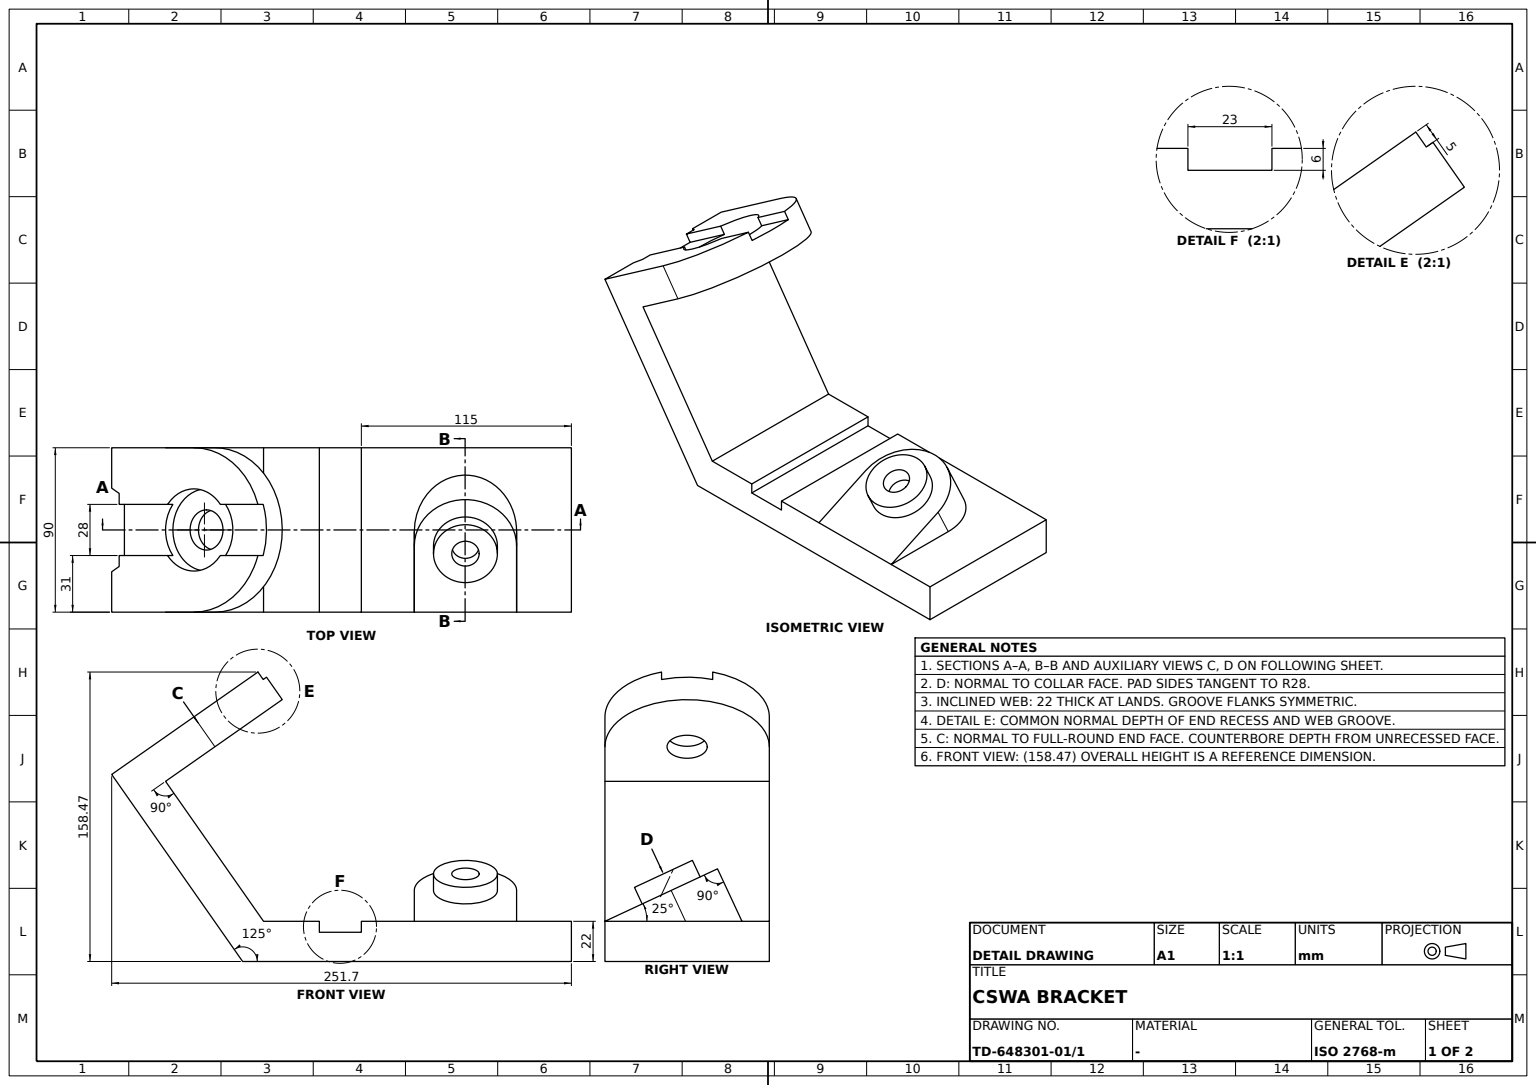
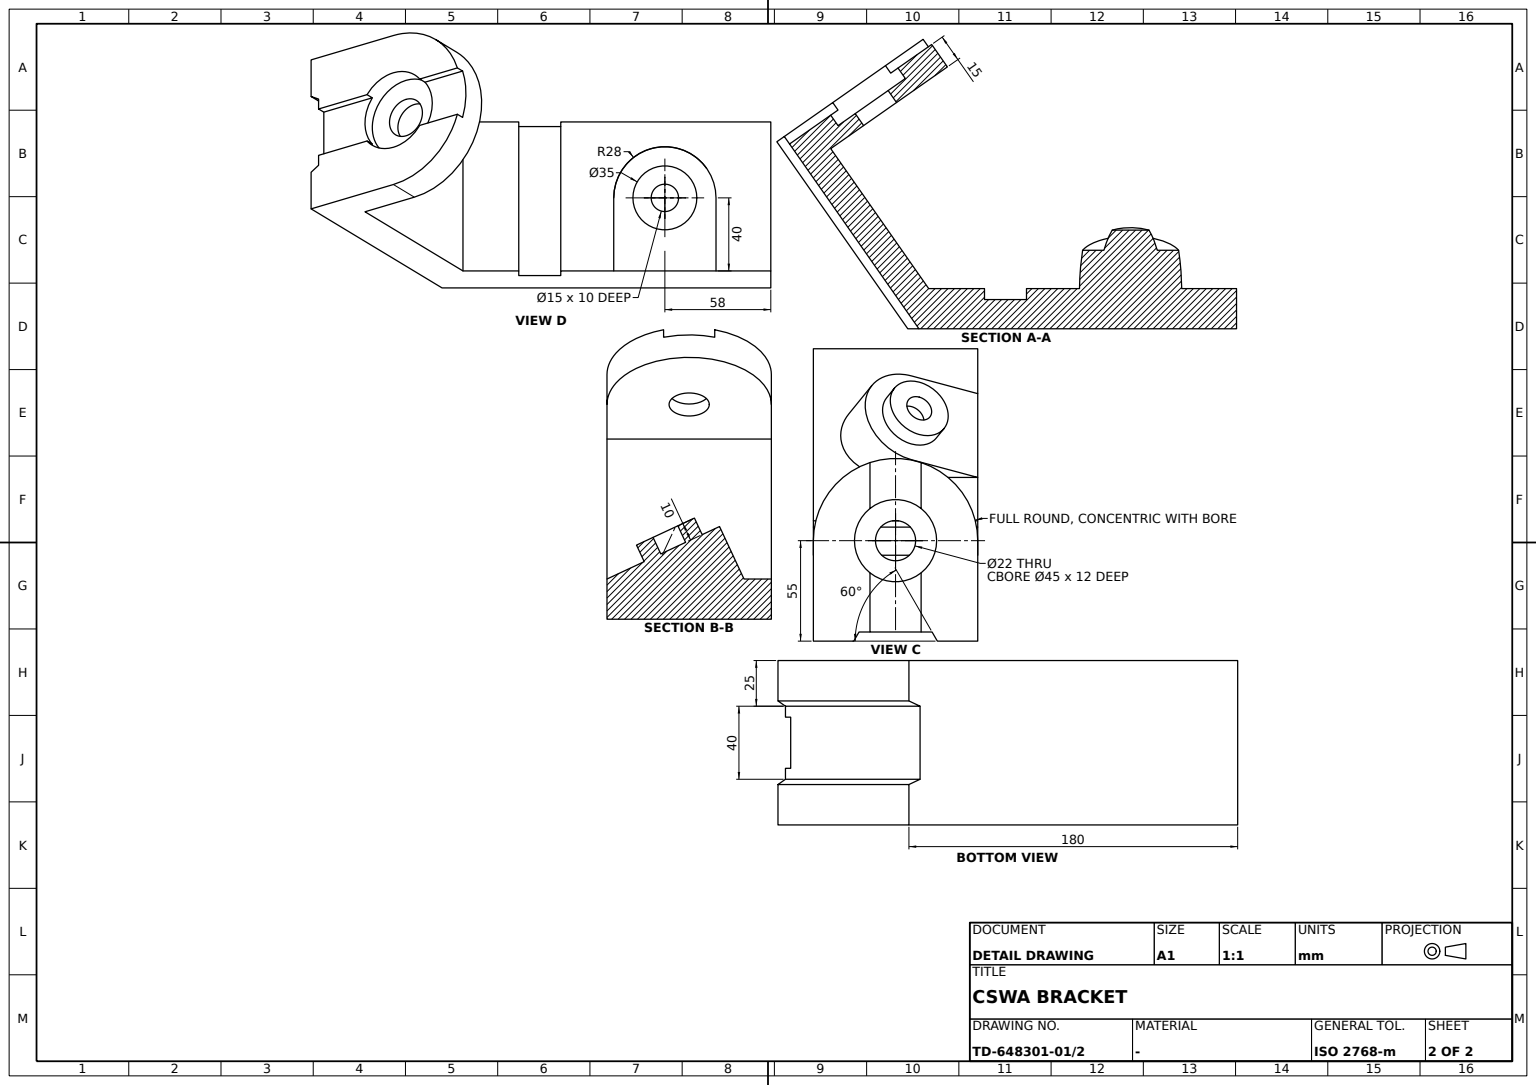
ISO-10303-21;
HEADER;
FILE_DESCRIPTION((''),'2;1');
FILE_NAME('','',(''),(''),'','','');
FILE_SCHEMA(('AUTOMOTIVE_DESIGN'));
ENDSEC;
DATA;
#1=APPLICATION_CONTEXT('');
#2=PRODUCT_CONTEXT('',#1,'mechanical');
#3=PRODUCT('','','',(#2));
#4=PRODUCT_DEFINITION_FORMATION('','',#3);
#5=PRODUCT_DEFINITION_CONTEXT('',#1,'design');
#6=PRODUCT_DEFINITION('','',#4,#5);
#7=PRODUCT_DEFINITION_SHAPE('','',#6);
#8=(LENGTH_UNIT()NAMED_UNIT(*)SI_UNIT(.MILLI.,.METRE.));
#9=(NAMED_UNIT(*)PLANE_ANGLE_UNIT()SI_UNIT($,.RADIAN.));
#10=(NAMED_UNIT(*)SI_UNIT($,.STERADIAN.)SOLID_ANGLE_UNIT());
#11=UNCERTAINTY_MEASURE_WITH_UNIT(LENGTH_MEASURE(1.E-05),#8,'distance_accuracy_value','');
#12=(GEOMETRIC_REPRESENTATION_CONTEXT(3)GLOBAL_UNCERTAINTY_ASSIGNED_CONTEXT((#11))GLOBAL_UNIT_ASSIGNED_CONTEXT((#8,#9,#10))REPRESENTATION_CONTEXT('',''));
#13=CARTESIAN_POINT('',(14.,11.25671,154.374984));
#14=VERTEX_POINT('',#13);
#15=CARTESIAN_POINT('',(-14.,11.25671,154.374984));
#16=VERTEX_POINT('',#15);
#17=CARTESIAN_POINT('',(0.,-23.77581,129.844949));
#18=DIRECTION('',(0.,-0.573576436,0.819152044));
#19=DIRECTION('',(1.,0.,0.));
#20=AXIS2_PLACEMENT_3D('',#17,#18,#19);
#21=CIRCLE('',#20,45.);
#22=EDGE_CURVE('',#14,#16,#21,.T.);
#23=ORIENTED_EDGE('',*,*,#22,.F.);
#24=CARTESIAN_POINT('',(14.,8.388827,158.470744));
#25=VERTEX_POINT('',#24);
#26=CARTESIAN_POINT('',(14.,9.822768,156.422864));
#27=DIRECTION('',(0.,0.573576436,-0.819152044));
#28=VECTOR('',#27,1000.);
#29=LINE('',#26,#28);
#30=EDGE_CURVE('',#25,#14,#29,.T.);
#31=ORIENTED_EDGE('',*,*,#30,.F.);
#32=CARTESIAN_POINT('',(45.,-26.643692,133.94071));
#33=VERTEX_POINT('',#32);
#34=CARTESIAN_POINT('',(0.,-26.643692,133.94071));
#35=AXIS2_PLACEMENT_3D('',#34,#18,#19);
#36=CIRCLE('',#35,45.);
#37=EDGE_CURVE('',#33,#25,#36,.T.);
#38=ORIENTED_EDGE('',*,*,#37,.F.);
#39=CARTESIAN_POINT('',(45.,-15.172163,117.557669));
#40=VERTEX_POINT('',#39);
#41=CARTESIAN_POINT('',(45.,-20.907928,125.749189));
#42=VECTOR('',#18,1000.);
#43=LINE('',#41,#42);
#44=EDGE_CURVE('',#40,#33,#43,.T.);
#45=ORIENTED_EDGE('',*,*,#44,.F.);
#46=CARTESIAN_POINT('',(-45.,-15.172163,117.557669));
#47=VERTEX_POINT('',#46);
#48=CARTESIAN_POINT('',(0.,-15.172163,117.557669));
#49=AXIS2_PLACEMENT_3D('',#48,#18,#19);
#50=CIRCLE('',#49,45.);
#51=EDGE_CURVE('',#40,#47,#50,.T.);
#52=ORIENTED_EDGE('',*,*,#51,.T.);
#53=CARTESIAN_POINT('',(-45.,-26.643692,133.94071));
#54=VERTEX_POINT('',#53);
#55=CARTESIAN_POINT('',(-45.,-20.907928,125.749189));
#56=LINE('',#55,#42);
#57=EDGE_CURVE('',#47,#54,#56,.T.);
#58=ORIENTED_EDGE('',*,*,#57,.T.);
#59=CARTESIAN_POINT('',(-14.,8.388827,158.470744));
#60=VERTEX_POINT('',#59);
#61=EDGE_CURVE('',#60,#54,#36,.T.);
#62=ORIENTED_EDGE('',*,*,#61,.F.);
#63=CARTESIAN_POINT('',(-14.,9.822768,156.422864));
#64=LINE('',#63,#28);
#65=EDGE_CURVE('',#60,#16,#64,.T.);
#66=ORIENTED_EDGE('',*,*,#65,.T.);
#67=EDGE_LOOP('',(#23,#31,#38,#45,#52,#58,#62,#66));
#68=FACE_OUTER_BOUND('',#67,.T.);
#69=CARTESIAN_POINT('',(0.,-20.907928,125.749189));
#70=AXIS2_PLACEMENT_3D('',#69,#27,#19);
#71=CYLINDRICAL_SURFACE('',#70,45.);
#72=ADVANCED_FACE('',(#68),#71,.T.);
#73=CARTESIAN_POINT('',(-14.,-38.204284,119.742023));
#74=VERTEX_POINT('',#73);
#75=CARTESIAN_POINT('',(14.,-38.204284,119.742023));
#76=VERTEX_POINT('',#75);
#77=CIRCLE('',#20,22.5);
#78=EDGE_CURVE('',#74,#76,#77,.T.);
#79=ORIENTED_EDGE('',*,*,#78,.F.);
#80=CARTESIAN_POINT('',(-14.,-64.733412,101.166127));
#81=VERTEX_POINT('',#80);
#82=CARTESIAN_POINT('',(-14.,-51.468848,110.454075));
#83=DIRECTION('',(0.,-0.819152044,-0.573576436));
#84=VECTOR('',#83,1000.);
#85=LINE('',#82,#84);
#86=EDGE_CURVE('',#74,#81,#85,.T.);
#87=ORIENTED_EDGE('',*,*,#86,.T.);
#88=CARTESIAN_POINT('',(14.,-64.733412,101.166127));
#89=VERTEX_POINT('',#88);
#90=CARTESIAN_POINT('',(0.,-64.733412,101.166127));
#91=VECTOR('',#19,1000.);
#92=LINE('',#90,#91);
#93=EDGE_CURVE('',#81,#89,#92,.T.);
#94=ORIENTED_EDGE('',*,*,#93,.T.);
#95=CARTESIAN_POINT('',(14.,-51.468848,110.454075));
#96=DIRECTION('',(0.,0.819152044,0.573576436));
#97=VECTOR('',#96,1000.);
#98=LINE('',#95,#97);
#99=EDGE_CURVE('',#89,#76,#98,.T.);
#100=ORIENTED_EDGE('',*,*,#99,.T.);
#101=EDGE_LOOP('',(#79,#87,#94,#100));
#102=FACE_OUTER_BOUND('',#101,.T.);
#103=CARTESIAN_POINT('',(0.,-68.829172,98.298245));
#104=AXIS2_PLACEMENT_3D('',#103,#18,#19);
#105=PLANE('',#104);
#106=ADVANCED_FACE('',(#102),#105,.T.);
#107=CARTESIAN_POINT('',(11.,-15.172163,117.557669));
#108=VERTEX_POINT('',#107);
#109=CARTESIAN_POINT('',(11.,-19.760775,124.110885));
#110=VERTEX_POINT('',#109);
#111=CARTESIAN_POINT('',(11.,-17.466469,120.834277));
#112=LINE('',#111,#42);
#113=EDGE_CURVE('',#108,#110,#112,.T.);
#114=ORIENTED_EDGE('',*,*,#113,.F.);
#115=CARTESIAN_POINT('',(-11.,-15.172163,117.557669));
#116=VERTEX_POINT('',#115);
#117=AXIS2_PLACEMENT_3D('',#48,#27,#19);
#118=CIRCLE('',#117,11.);
#119=EDGE_CURVE('',#108,#116,#118,.T.);
#120=ORIENTED_EDGE('',*,*,#119,.T.);
#121=CARTESIAN_POINT('',(-11.,-19.760775,124.110885));
#122=VERTEX_POINT('',#121);
#123=CARTESIAN_POINT('',(-11.,-17.466469,120.834277));
#124=LINE('',#123,#42);
#125=EDGE_CURVE('',#116,#122,#124,.T.);
#126=ORIENTED_EDGE('',*,*,#125,.T.);
#127=CARTESIAN_POINT('',(0.,-19.760775,124.110885));
#128=AXIS2_PLACEMENT_3D('',#127,#27,#19);
#129=CIRCLE('',#128,11.);
#130=EDGE_CURVE('',#110,#122,#129,.T.);
#131=ORIENTED_EDGE('',*,*,#130,.F.);
#132=EDGE_LOOP('',(#114,#120,#126,#131));
#133=FACE_OUTER_BOUND('',#132,.T.);
#134=CYLINDRICAL_SURFACE('',#35,11.);
#135=ADVANCED_FACE('',(#133),#134,.F.);
#136=CARTESIAN_POINT('',(45.,42.,22.));
#137=VERTEX_POINT('',#136);
#138=CARTESIAN_POINT('',(45.,11.452475,22.));
#139=VERTEX_POINT('',#138);
#140=CARTESIAN_POINT('',(45.,26.726238,22.));
#141=DIRECTION('',(0.,-1.,0.));
#142=VECTOR('',#141,1000.);
#143=LINE('',#140,#142);
#144=EDGE_CURVE('',#137,#139,#143,.T.);
#145=ORIENTED_EDGE('',*,*,#144,.F.);
#146=CARTESIAN_POINT('',(-45.,42.,22.));
#147=VERTEX_POINT('',#146);
#148=CARTESIAN_POINT('',(0.,42.,22.));
#149=LINE('',#148,#91);
#150=EDGE_CURVE('',#147,#137,#149,.T.);
#151=ORIENTED_EDGE('',*,*,#150,.F.);
#152=CARTESIAN_POINT('',(-45.,11.452475,22.));
#153=VERTEX_POINT('',#152);
#154=CARTESIAN_POINT('',(-45.,26.726238,22.));
#155=LINE('',#154,#142);
#156=EDGE_CURVE('',#147,#153,#155,.T.);
#157=ORIENTED_EDGE('',*,*,#156,.T.);
#158=CARTESIAN_POINT('',(0.,11.452475,22.));
#159=LINE('',#158,#91);
#160=EDGE_CURVE('',#153,#139,#159,.T.);
#161=ORIENTED_EDGE('',*,*,#160,.T.);
#162=EDGE_LOOP('',(#145,#151,#157,#161));
#163=FACE_OUTER_BOUND('',#162,.T.);
#164=CARTESIAN_POINT('',(0.,65.,22.));
#165=DIRECTION('',(0.,0.,-1.));
#166=DIRECTION('',(0.,1.,0.));
#167=AXIS2_PLACEMENT_3D('',#164,#165,#166);
#168=PLANE('',#167);
#169=ADVANCED_FACE('',(#163),#168,.F.);
#170=CARTESIAN_POINT('',(-45.,0.,0.));
#171=VERTEX_POINT('',#170);
#172=CARTESIAN_POINT('',(-45.,180.,0.));
#173=VERTEX_POINT('',#172);
#174=CARTESIAN_POINT('',(-45.,90.,0.));
#175=VECTOR('',#166,1000.);
#176=LINE('',#174,#175);
#177=EDGE_CURVE('',#171,#173,#176,.T.);
#178=ORIENTED_EDGE('',*,*,#177,.F.);
#179=CARTESIAN_POINT('',(-45.,-71.697055,102.394006));
#180=VERTEX_POINT('',#179);
#181=CARTESIAN_POINT('',(-45.,-35.848527,51.197003));
#182=LINE('',#181,#28);
#183=EDGE_CURVE('',#180,#171,#182,.T.);
#184=ORIENTED_EDGE('',*,*,#183,.F.);
#185=CARTESIAN_POINT('',(-45.,-49.170373,118.167358));
#186=LINE('',#185,#84);
#187=EDGE_CURVE('',#54,#180,#186,.T.);
#188=ORIENTED_EDGE('',*,*,#187,.F.);
#189=ORIENTED_EDGE('',*,*,#57,.F.);
#190=CARTESIAN_POINT('',(-45.,-42.204181,98.629646));
#191=VERTEX_POINT('',#190);
#192=CARTESIAN_POINT('',(-45.,-28.688172,108.093657));
#193=LINE('',#192,#97);
#194=EDGE_CURVE('',#191,#47,#193,.T.);
#195=ORIENTED_EDGE('',*,*,#194,.F.);
#196=CARTESIAN_POINT('',(-45.,-15.375853,60.314823));
#197=LINE('',#196,#42);
#198=EDGE_CURVE('',#153,#191,#197,.T.);
#199=ORIENTED_EDGE('',*,*,#198,.F.);
#200=ORIENTED_EDGE('',*,*,#156,.F.);
#201=CARTESIAN_POINT('',(-45.,42.,16.));
#202=VERTEX_POINT('',#201);
#203=CARTESIAN_POINT('',(-45.,42.,19.));
#204=DIRECTION('',(0.,0.,1.));
#205=VECTOR('',#204,1000.);
#206=LINE('',#203,#205);
#207=EDGE_CURVE('',#202,#147,#206,.T.);
#208=ORIENTED_EDGE('',*,*,#207,.F.);
#209=CARTESIAN_POINT('',(-45.,65.,16.));
#210=VERTEX_POINT('',#209);
#211=CARTESIAN_POINT('',(-45.,53.5,16.));
#212=LINE('',#211,#142);
#213=EDGE_CURVE('',#210,#202,#212,.T.);
#214=ORIENTED_EDGE('',*,*,#213,.F.);
#215=CARTESIAN_POINT('',(-45.,65.,22.));
#216=VERTEX_POINT('',#215);
#217=CARTESIAN_POINT('',(-45.,65.,19.));
#218=VECTOR('',#165,1000.);
#219=LINE('',#217,#218);
#220=EDGE_CURVE('',#216,#210,#219,.T.);
#221=ORIENTED_EDGE('',*,*,#220,.F.);
#222=CARTESIAN_POINT('',(-45.,180.,22.));
#223=VERTEX_POINT('',#222);
#224=CARTESIAN_POINT('',(-45.,122.5,22.));
#225=LINE('',#224,#142);
#226=EDGE_CURVE('',#223,#216,#225,.T.);
#227=ORIENTED_EDGE('',*,*,#226,.F.);
#228=CARTESIAN_POINT('',(-45.,180.,11.));
#229=LINE('',#228,#205);
#230=EDGE_CURVE('',#173,#223,#229,.T.);
#231=ORIENTED_EDGE('',*,*,#230,.F.);
#232=EDGE_LOOP('',(#178,#184,#188,#189,#195,#199,#200,#208,#214,#221,#227,#231));
#233=FACE_OUTER_BOUND('',#232,.T.);
#234=AXIS2_PLACEMENT_3D('',#170,#19,#166);
#235=PLANE('',#234);
#236=ADVANCED_FACE('',(#233),#235,.F.);
#237=ORIENTED_EDGE('',*,*,#220,.T.);
#238=CARTESIAN_POINT('',(45.,65.,16.));
#239=VERTEX_POINT('',#238);
#240=CARTESIAN_POINT('',(0.,65.,16.));
#241=LINE('',#240,#91);
#242=EDGE_CURVE('',#210,#239,#241,.T.);
#243=ORIENTED_EDGE('',*,*,#242,.T.);
#244=CARTESIAN_POINT('',(45.,65.,22.));
#245=VERTEX_POINT('',#244);
#246=CARTESIAN_POINT('',(45.,65.,19.));
#247=LINE('',#246,#218);
#248=EDGE_CURVE('',#245,#239,#247,.T.);
#249=ORIENTED_EDGE('',*,*,#248,.F.);
#250=LINE('',#164,#91);
#251=EDGE_CURVE('',#216,#245,#250,.T.);
#252=ORIENTED_EDGE('',*,*,#251,.F.);
#253=EDGE_LOOP('',(#237,#243,#249,#252));
#254=FACE_OUTER_BOUND('',#253,.T.);
#255=AXIS2_PLACEMENT_3D('',#240,#166,#204);
#256=PLANE('',#255);
#257=ADVANCED_FACE('',(#254),#256,.F.);
#258=CARTESIAN_POINT('',(45.,150.,22.));
#259=VERTEX_POINT('',#258);
#260=CARTESIAN_POINT('',(45.,94.,22.));
#261=VERTEX_POINT('',#260);
#262=CARTESIAN_POINT('',(45.,122.,22.));
#263=LINE('',#262,#142);
#264=EDGE_CURVE('',#259,#261,#263,.T.);
#265=ORIENTED_EDGE('',*,*,#264,.T.);
#266=CARTESIAN_POINT('',(45.,79.5,22.));
#267=LINE('',#266,#142);
#268=EDGE_CURVE('',#261,#245,#267,.T.);
#269=ORIENTED_EDGE('',*,*,#268,.T.);
#270=ORIENTED_EDGE('',*,*,#248,.T.);
#271=CARTESIAN_POINT('',(45.,42.,16.));
#272=VERTEX_POINT('',#271);
#273=CARTESIAN_POINT('',(45.,53.5,16.));
#274=LINE('',#273,#142);
#275=EDGE_CURVE('',#239,#272,#274,.T.);
#276=ORIENTED_EDGE('',*,*,#275,.T.);
#277=CARTESIAN_POINT('',(45.,42.,19.));
#278=LINE('',#277,#205);
#279=EDGE_CURVE('',#272,#137,#278,.T.);
#280=ORIENTED_EDGE('',*,*,#279,.T.);
#281=ORIENTED_EDGE('',*,*,#144,.T.);
#282=CARTESIAN_POINT('',(45.,-42.204181,98.629646));
#283=VERTEX_POINT('',#282);
#284=CARTESIAN_POINT('',(45.,-15.375853,60.314823));
#285=LINE('',#284,#42);
#286=EDGE_CURVE('',#139,#283,#285,.T.);
#287=ORIENTED_EDGE('',*,*,#286,.T.);
#288=CARTESIAN_POINT('',(45.,-28.688172,108.093657));
#289=LINE('',#288,#97);
#290=EDGE_CURVE('',#283,#40,#289,.T.);
#291=ORIENTED_EDGE('',*,*,#290,.T.);
#292=ORIENTED_EDGE('',*,*,#44,.T.);
#293=CARTESIAN_POINT('',(45.,-71.697055,102.394006));
#294=VERTEX_POINT('',#293);
#295=CARTESIAN_POINT('',(45.,-49.170373,118.167358));
#296=LINE('',#295,#84);
#297=EDGE_CURVE('',#33,#294,#296,.T.);
#298=ORIENTED_EDGE('',*,*,#297,.T.);
#299=CARTESIAN_POINT('',(45.,0.,0.));
#300=VERTEX_POINT('',#299);
#301=CARTESIAN_POINT('',(45.,-35.848527,51.197003));
#302=LINE('',#301,#28);
#303=EDGE_CURVE('',#294,#300,#302,.T.);
#304=ORIENTED_EDGE('',*,*,#303,.T.);
#305=CARTESIAN_POINT('',(45.,180.,0.));
#306=VERTEX_POINT('',#305);
#307=CARTESIAN_POINT('',(45.,90.,0.));
#308=LINE('',#307,#175);
#309=EDGE_CURVE('',#300,#306,#308,.T.);
#310=ORIENTED_EDGE('',*,*,#309,.T.);
#311=CARTESIAN_POINT('',(45.,180.,22.));
#312=VERTEX_POINT('',#311);
#313=CARTESIAN_POINT('',(45.,180.,11.));
#314=LINE('',#313,#205);
#315=EDGE_CURVE('',#306,#312,#314,.T.);
#316=ORIENTED_EDGE('',*,*,#315,.T.);
#317=CARTESIAN_POINT('',(45.,165.,22.));
#318=LINE('',#317,#142);
#319=EDGE_CURVE('',#312,#259,#318,.T.);
#320=ORIENTED_EDGE('',*,*,#319,.T.);
#321=EDGE_LOOP('',(#265,#269,#270,#276,#280,#281,#287,#291,#292,#298,#304,#310,#316,#320));
#322=FACE_OUTER_BOUND('',#321,.T.);
#323=AXIS2_PLACEMENT_3D('',#299,#19,#166);
#324=PLANE('',#323);
#325=ADVANCED_FACE('',(#322),#324,.T.);
#326=CARTESIAN_POINT('',(-22.886751,0.,0.));
#327=VERTEX_POINT('',#326);
#328=CARTESIAN_POINT('',(-33.943376,0.,0.));
#329=LINE('',#328,#91);
#330=EDGE_CURVE('',#171,#327,#329,.T.);
#331=ORIENTED_EDGE('',*,*,#330,.T.);
#332=CARTESIAN_POINT('',(-22.886751,-71.697055,102.394006));
#333=VERTEX_POINT('',#332);
#334=CARTESIAN_POINT('',(-22.886751,-35.848527,51.197003));
#335=LINE('',#334,#28);
#336=EDGE_CURVE('',#333,#327,#335,.T.);
#337=ORIENTED_EDGE('',*,*,#336,.F.);
#338=CARTESIAN_POINT('',(-33.943376,-71.697055,102.394006));
#339=LINE('',#338,#91);
#340=EDGE_CURVE('',#180,#333,#339,.T.);
#341=ORIENTED_EDGE('',*,*,#340,.F.);
#342=ORIENTED_EDGE('',*,*,#183,.T.);
#343=EDGE_LOOP('',(#331,#337,#341,#342));
#344=FACE_OUTER_BOUND('',#343,.T.);
#345=CARTESIAN_POINT('',(0.,0.,0.));
#346=AXIS2_PLACEMENT_3D('',#345,#96,#18);
#347=PLANE('',#346);
#348=ADVANCED_FACE('',(#344),#347,.F.);
#349=ORIENTED_EDGE('',*,*,#297,.F.);
#350=ORIENTED_EDGE('',*,*,#37,.T.);
#351=CARTESIAN_POINT('',(14.,-12.215218,144.043636));
#352=VERTEX_POINT('',#351);
#353=CARTESIAN_POINT('',(14.,-1.913195,151.25719));
#354=LINE('',#353,#97);
#355=EDGE_CURVE('',#352,#25,#354,.T.);
#356=ORIENTED_EDGE('',*,*,#355,.F.);
#357=CARTESIAN_POINT('',(22.5,-26.643692,133.94071));
#358=VERTEX_POINT('',#357);
#359=AXIS2_PLACEMENT_3D('',#34,#27,#96);
#360=CIRCLE('',#359,22.5);
#361=EDGE_CURVE('',#352,#358,#360,.T.);
#362=ORIENTED_EDGE('',*,*,#361,.T.);
#363=CARTESIAN_POINT('',(14.,-41.072167,123.837783));
#364=VERTEX_POINT('',#363);
#365=EDGE_CURVE('',#358,#364,#360,.T.);
#366=ORIENTED_EDGE('',*,*,#365,.T.);
#367=CARTESIAN_POINT('',(14.,-67.601294,105.261888));
#368=VERTEX_POINT('',#367);
#369=CARTESIAN_POINT('',(14.,-54.33673,114.549835));
#370=LINE('',#369,#97);
#371=EDGE_CURVE('',#368,#364,#370,.T.);
#372=ORIENTED_EDGE('',*,*,#371,.F.);
#373=CARTESIAN_POINT('',(20.,-67.601294,105.261888));
#374=VERTEX_POINT('',#373);
#375=CARTESIAN_POINT('',(17.,-67.601294,105.261888));
#376=DIRECTION('',(-1.,0.,0.));
#377=VECTOR('',#376,1000.);
#378=LINE('',#375,#377);
#379=EDGE_CURVE('',#374,#368,#378,.T.);
#380=ORIENTED_EDGE('',*,*,#379,.F.);
#381=CARTESIAN_POINT('',(22.886751,-71.697055,102.394006));
#382=VERTEX_POINT('',#381);
#383=CARTESIAN_POINT('',(21.443376,-69.649174,103.827947));
#384=DIRECTION('',(-0.5,0.70940648,0.496731765));
#385=VECTOR('',#384,1000.);
#386=LINE('',#383,#385);
#387=EDGE_CURVE('',#382,#374,#386,.T.);
#388=ORIENTED_EDGE('',*,*,#387,.F.);
#389=CARTESIAN_POINT('',(33.943376,-71.697055,102.394006));
#390=LINE('',#389,#91);
#391=EDGE_CURVE('',#382,#294,#390,.T.);
#392=ORIENTED_EDGE('',*,*,#391,.T.);
#393=EDGE_LOOP('',(#349,#350,#356,#362,#366,#372,#380,#388,#392));
#394=FACE_OUTER_BOUND('',#393,.T.);
#395=CARTESIAN_POINT('',(0.,-71.697055,102.394006));
#396=AXIS2_PLACEMENT_3D('',#395,#27,#96);
#397=PLANE('',#396);
#398=ADVANCED_FACE('',(#394),#397,.F.);
#399=CARTESIAN_POINT('',(8.747689,139.5,38.90473));
#400=VERTEX_POINT('',#399);
#401=CARTESIAN_POINT('',(12.973871,139.5,47.967808));
#402=VERTEX_POINT('',#401);
#403=CARTESIAN_POINT('',(10.86078,139.5,43.436269));
#404=DIRECTION('',(0.422618262,0.,0.906307787));
#405=VECTOR('',#404,1000.);
#406=LINE('',#403,#405);
#407=EDGE_CURVE('',#400,#402,#406,.T.);
#408=ORIENTED_EDGE('',*,*,#407,.T.);
#409=CARTESIAN_POINT('',(12.973871,104.5,47.967808));
#410=VERTEX_POINT('',#409);
#411=CARTESIAN_POINT('',(12.973871,122.,47.967808));
#412=AXIS2_PLACEMENT_3D('',#411,#404,#166);
#413=CIRCLE('',#412,17.5);
#414=EDGE_CURVE('',#410,#402,#413,.T.);
#415=ORIENTED_EDGE('',*,*,#414,.F.);
#416=CARTESIAN_POINT('',(8.747689,104.5,38.90473));
#417=VERTEX_POINT('',#416);
#418=CARTESIAN_POINT('',(10.86078,104.5,43.436269));
#419=LINE('',#418,#405);
#420=EDGE_CURVE('',#417,#410,#419,.T.);
#421=ORIENTED_EDGE('',*,*,#420,.F.);
#422=CARTESIAN_POINT('',(8.747689,122.,38.90473));
#423=AXIS2_PLACEMENT_3D('',#422,#404,#166);
#424=CIRCLE('',#423,17.5);
#425=EDGE_CURVE('',#417,#400,#424,.T.);
#426=ORIENTED_EDGE('',*,*,#425,.T.);
#427=EDGE_LOOP('',(#408,#415,#421,#426));
#428=FACE_OUTER_BOUND('',#427,.T.);
#429=CARTESIAN_POINT('',(10.86078,122.,43.436269));
#430=DIRECTION('',(-0.422618262,0.,-0.906307787));
#431=AXIS2_PLACEMENT_3D('',#429,#430,#166);
#432=CYLINDRICAL_SURFACE('',#431,17.5);
#433=ADVANCED_FACE('',(#428),#432,.T.);
#434=CARTESIAN_POINT('',(-14.,-41.072167,123.837783));
#435=VERTEX_POINT('',#434);
#436=CARTESIAN_POINT('',(-14.,-67.601294,105.261888));
#437=VERTEX_POINT('',#436);
#438=CARTESIAN_POINT('',(-14.,-54.33673,114.549835));
#439=LINE('',#438,#84);
#440=EDGE_CURVE('',#435,#437,#439,.T.);
#441=ORIENTED_EDGE('',*,*,#440,.T.);
#442=CARTESIAN_POINT('',(-14.,-66.167353,103.214008));
#443=LINE('',#442,#28);
#444=EDGE_CURVE('',#437,#81,#443,.T.);
#445=ORIENTED_EDGE('',*,*,#444,.T.);
#446=ORIENTED_EDGE('',*,*,#86,.F.);
#447=CARTESIAN_POINT('',(-14.,-39.638225,121.789903));
#448=LINE('',#447,#28);
#449=EDGE_CURVE('',#435,#74,#448,.T.);
#450=ORIENTED_EDGE('',*,*,#449,.F.);
#451=EDGE_LOOP('',(#441,#445,#446,#450));
#452=FACE_OUTER_BOUND('',#451,.T.);
#453=CARTESIAN_POINT('',(-14.,-103.880285,79.859065));
#454=AXIS2_PLACEMENT_3D('',#453,#376,#96);
#455=PLANE('',#454);
#456=ADVANCED_FACE('',(#452),#455,.F.);
#457=CARTESIAN_POINT('',(14.,-39.638225,121.789903));
#458=LINE('',#457,#28);
#459=EDGE_CURVE('',#364,#76,#458,.T.);
#460=ORIENTED_EDGE('',*,*,#459,.T.);
#461=ORIENTED_EDGE('',*,*,#99,.F.);
#462=CARTESIAN_POINT('',(14.,-66.167353,103.214008));
#463=LINE('',#462,#28);
#464=EDGE_CURVE('',#368,#89,#463,.T.);
#465=ORIENTED_EDGE('',*,*,#464,.F.);
#466=ORIENTED_EDGE('',*,*,#371,.T.);
#467=EDGE_LOOP('',(#460,#461,#465,#466));
#468=FACE_OUTER_BOUND('',#467,.T.);
#469=CARTESIAN_POINT('',(14.,16.525409,164.168039));
#470=AXIS2_PLACEMENT_3D('',#469,#19,#83);
#471=PLANE('',#470);
#472=ADVANCED_FACE('',(#468),#471,.F.);
#473=CARTESIAN_POINT('',(8.747689,114.5,38.90473));
#474=VERTEX_POINT('',#473);
#475=CARTESIAN_POINT('',(8.747689,129.5,38.90473));
#476=VERTEX_POINT('',#475);
#477=CIRCLE('',#423,7.5);
#478=EDGE_CURVE('',#474,#476,#477,.T.);
#479=ORIENTED_EDGE('',*,*,#478,.T.);
#480=EDGE_CURVE('',#476,#474,#477,.T.);
#481=ORIENTED_EDGE('',*,*,#480,.T.);
#482=EDGE_LOOP('',(#479,#481));
#483=FACE_OUTER_BOUND('',#482,.T.);
#484=CARTESIAN_POINT('',(16.463768,0.,35.306664));
#485=AXIS2_PLACEMENT_3D('',#484,#430,#141);
#486=PLANE('',#485);
#487=ADVANCED_FACE('',(#483),#486,.F.);
#488=ORIENTED_EDGE('',*,*,#242,.F.);
#489=ORIENTED_EDGE('',*,*,#213,.T.);
#490=CARTESIAN_POINT('',(0.,42.,16.));
#491=LINE('',#490,#91);
#492=EDGE_CURVE('',#202,#272,#491,.T.);
#493=ORIENTED_EDGE('',*,*,#492,.T.);
#494=ORIENTED_EDGE('',*,*,#275,.F.);
#495=EDGE_LOOP('',(#488,#489,#493,#494));
#496=FACE_OUTER_BOUND('',#495,.T.);
#497=AXIS2_PLACEMENT_3D('',#490,#165,#166);
#498=PLANE('',#497);
#499=ADVANCED_FACE('',(#496),#498,.F.);
#500=ORIENTED_EDGE('',*,*,#365,.F.);
#501=CARTESIAN_POINT('',(22.5,-19.760775,124.110885));
#502=VERTEX_POINT('',#501);
#503=CARTESIAN_POINT('',(22.5,-36.778166,148.414238));
#504=LINE('',#503,#42);
#505=EDGE_CURVE('',#502,#358,#504,.T.);
#506=ORIENTED_EDGE('',*,*,#505,.F.);
#507=CARTESIAN_POINT('',(-22.5,-19.760775,124.110885));
#508=VERTEX_POINT('',#507);
#509=CIRCLE('',#128,22.5);
#510=EDGE_CURVE('',#502,#508,#509,.T.);
#511=ORIENTED_EDGE('',*,*,#510,.T.);
#512=CARTESIAN_POINT('',(-22.5,-26.643692,133.94071));
#513=VERTEX_POINT('',#512);
#514=CARTESIAN_POINT('',(-22.5,-36.778166,148.414238));
#515=LINE('',#514,#42);
#516=EDGE_CURVE('',#508,#513,#515,.T.);
#517=ORIENTED_EDGE('',*,*,#516,.T.);
#518=EDGE_CURVE('',#435,#513,#360,.T.);
#519=ORIENTED_EDGE('',*,*,#518,.F.);
#520=ORIENTED_EDGE('',*,*,#449,.T.);
#521=ORIENTED_EDGE('',*,*,#78,.T.);
#522=ORIENTED_EDGE('',*,*,#459,.F.);
#523=EDGE_LOOP('',(#500,#506,#511,#517,#519,#520,#521,#522));
#524=FACE_OUTER_BOUND('',#523,.T.);
#525=CYLINDRICAL_SURFACE('',#35,22.5);
#526=ADVANCED_FACE('',(#524),#525,.F.);
#527=CARTESIAN_POINT('',(20.,6.103873,0.));
#528=VERTEX_POINT('',#527);
#529=CARTESIAN_POINT('',(20.,-30.748711,52.630944));
#530=LINE('',#529,#28);
#531=EDGE_CURVE('',#374,#528,#530,.T.);
#532=ORIENTED_EDGE('',*,*,#531,.T.);
#533=CARTESIAN_POINT('',(22.886751,0.,0.));
#534=VERTEX_POINT('',#533);
#535=CARTESIAN_POINT('',(21.443376,3.051936,0.));
#536=DIRECTION('',(-0.427535057,0.90399877,0.));
#537=VECTOR('',#536,1000.);
#538=LINE('',#535,#537);
#539=EDGE_CURVE('',#534,#528,#538,.T.);
#540=ORIENTED_EDGE('',*,*,#539,.F.);
#541=CARTESIAN_POINT('',(22.886751,-35.848527,51.197003));
#542=LINE('',#541,#28);
#543=EDGE_CURVE('',#382,#534,#542,.T.);
#544=ORIENTED_EDGE('',*,*,#543,.F.);
#545=ORIENTED_EDGE('',*,*,#387,.T.);
#546=EDGE_LOOP('',(#532,#540,#544,#545));
#547=FACE_OUTER_BOUND('',#546,.T.);
#548=DIRECTION('',(0.866025404,0.409576022,0.286788218));
#549=DIRECTION('',(0.5,-0.70940648,-0.496731765));
#550=AXIS2_PLACEMENT_3D('',#373,#548,#549);
#551=PLANE('',#550);
#552=ADVANCED_FACE('',(#547),#551,.F.);
#553=CARTESIAN_POINT('',(0.864883,94.,22.));
#554=VERTEX_POINT('',#553);
#555=CARTESIAN_POINT('',(0.864883,150.,22.));
#556=VERTEX_POINT('',#555);
#557=CARTESIAN_POINT('',(-1.788464,94.,22.));
#558=CARTESIAN_POINT('',(-4.441812,94.258162,22.));
#559=CARTESIAN_POINT('',(-7.062296,94.774522,22.));
#560=CARTESIAN_POINT('',(-11.709183,96.180854,22.));
#561=CARTESIAN_POINT('',(-16.010347,98.415099,22.));
#562=CARTESIAN_POINT('',(-17.85824,99.586628,22.));
#563=CARTESIAN_POINT('',(-21.220025,102.164081,22.));
#564=CARTESIAN_POINT('',(-24.070826,105.294522,22.));
#565=CARTESIAN_POINT('',(-25.312082,106.930022,22.));
#566=CARTESIAN_POINT('',(-27.421449,110.322656,22.));
#567=CARTESIAN_POINT('',(-28.869875,114.043793,22.));
#568=CARTESIAN_POINT('',(-29.404569,115.915462,22.));
#569=CARTESIAN_POINT('',(-30.13655,119.862177,22.));
#570=CARTESIAN_POINT('',(-30.086708,123.878297,22.));
#571=CARTESIAN_POINT('',(-29.849179,125.939472,22.));
#572=CARTESIAN_POINT('',(-28.984605,129.878622,22.));
#573=CARTESIAN_POINT('',(-27.384871,133.578503,22.));
#574=CARTESIAN_POINT('',(-26.443124,135.301263,22.));
#575=CARTESIAN_POINT('',(-24.201022,138.653542,22.));
#576=CARTESIAN_POINT('',(-21.402212,141.559699,22.));
#577=CARTESIAN_POINT('',(-19.83563,142.921994,22.));
#578=CARTESIAN_POINT('',(-16.382061,145.443221,22.));
#579=CARTESIAN_POINT('',(-12.550229,147.34504,22.));
#580=CARTESIAN_POINT('',(-10.497419,148.154241,22.));
#581=CARTESIAN_POINT('',(-7.01232,149.203696,22.));
#582=CARTESIAN_POINT('',(-3.424712,149.774537,22.));
#583=CARTESIAN_POINT('',(-1.998337,149.924846,22.));
#584=CARTESIAN_POINT('',(-0.566727,150.,22.));
#585=B_SPLINE_CURVE_WITH_KNOTS('',5,(#553,#557,#558,#559,#560,#561,#562,#563,#564,#565,#566,#567,#568,#569,#570,#571,#572,#573,#574,#575,#576,#577,#578,#579,#580,#581,#582,#583,#584,#555),.UNSPECIFIED.,.F.,.F.,(6,3,3,3,3,3,3,3,3,6),(0.,18.762001028,34.152888631,48.589777188,62.273886775,76.845629636,90.652395856,105.257427652,120.785414804,130.908425648),.UNSPECIFIED.);
#586=EDGE_CURVE('',#554,#556,#585,.T.);
#587=ORIENTED_EDGE('',*,*,#586,.F.);
#588=CARTESIAN_POINT('',(8.747689,94.,38.90473));
#589=VERTEX_POINT('',#588);
#590=CARTESIAN_POINT('',(4.806286,94.,30.452365));
#591=VECTOR('',#430,1000.);
#592=LINE('',#590,#591);
#593=EDGE_CURVE('',#589,#554,#592,.T.);
#594=ORIENTED_EDGE('',*,*,#593,.F.);
#595=CARTESIAN_POINT('',(8.747689,150.,38.90473));
#596=VERTEX_POINT('',#595);
#597=AXIS2_PLACEMENT_3D('',#422,#430,#141);
#598=CIRCLE('',#597,28.);
#599=EDGE_CURVE('',#589,#596,#598,.T.);
#600=ORIENTED_EDGE('',*,*,#599,.T.);
#601=CARTESIAN_POINT('',(-14.811313,150.,-11.617711));
#602=LINE('',#601,#591);
#603=EDGE_CURVE('',#596,#556,#602,.T.);
#604=ORIENTED_EDGE('',*,*,#603,.T.);
#605=EDGE_LOOP('',(#587,#594,#600,#604));
#606=FACE_OUTER_BOUND('',#605,.T.);
#607=CARTESIAN_POINT('',(-14.811313,122.,-11.617711));
#608=AXIS2_PLACEMENT_3D('',#607,#404,#141);
#609=CYLINDRICAL_SURFACE('',#608,28.);
#610=ADVANCED_FACE('',(#606),#609,.T.);
#611=AXIS2_PLACEMENT_3D('',#48,#27,#83);
#612=CIRCLE('',#611,11.);
#613=EDGE_CURVE('',#116,#108,#612,.T.);
#614=ORIENTED_EDGE('',*,*,#613,.F.);
#615=ORIENTED_EDGE('',*,*,#119,.F.);
#616=EDGE_LOOP('',(#614,#615));
#617=FACE_BOUND('',#616,.T.);
#618=ORIENTED_EDGE('',*,*,#290,.F.);
#619=CARTESIAN_POINT('',(0.,-42.204181,98.629646));
#620=LINE('',#619,#91);
#621=EDGE_CURVE('',#191,#283,#620,.T.);
#622=ORIENTED_EDGE('',*,*,#621,.F.);
#623=ORIENTED_EDGE('',*,*,#194,.T.);
#624=ORIENTED_EDGE('',*,*,#51,.F.);
#625=EDGE_LOOP('',(#618,#622,#623,#624));
#626=FACE_OUTER_BOUND('',#625,.T.);
#627=AXIS2_PLACEMENT_3D('',#48,#18,#83);
#628=PLANE('',#627);
#629=ADVANCED_FACE('',(#617,#626),#628,.F.);
#630=CARTESIAN_POINT('',(12.973871,114.5,47.967808));
#631=VERTEX_POINT('',#630);
#632=CARTESIAN_POINT('',(10.86078,114.5,43.436269));
#633=LINE('',#632,#591);
#634=EDGE_CURVE('',#631,#474,#633,.T.);
#635=ORIENTED_EDGE('',*,*,#634,.F.);
#636=CARTESIAN_POINT('',(12.973871,129.5,47.967808));
#637=VERTEX_POINT('',#636);
#638=CIRCLE('',#412,7.5);
#639=EDGE_CURVE('',#631,#637,#638,.T.);
#640=ORIENTED_EDGE('',*,*,#639,.T.);
#641=CARTESIAN_POINT('',(10.86078,129.5,43.436269));
#642=LINE('',#641,#591);
#643=EDGE_CURVE('',#637,#476,#642,.T.);
#644=ORIENTED_EDGE('',*,*,#643,.T.);
#645=ORIENTED_EDGE('',*,*,#478,.F.);
#646=EDGE_LOOP('',(#635,#640,#644,#645));
#647=FACE_OUTER_BOUND('',#646,.T.);
#648=CYLINDRICAL_SURFACE('',#431,7.5);
#649=ADVANCED_FACE('',(#647),#648,.F.);
#650=CARTESIAN_POINT('',(-20.,-67.601294,105.261888));
#651=VERTEX_POINT('',#650);
#652=CARTESIAN_POINT('',(-20.,6.103873,0.));
#653=VERTEX_POINT('',#652);
#654=CARTESIAN_POINT('',(-20.,-30.748711,52.630944));
#655=LINE('',#654,#28);
#656=EDGE_CURVE('',#651,#653,#655,.T.);
#657=ORIENTED_EDGE('',*,*,#656,.F.);
#658=CARTESIAN_POINT('',(-21.443376,-69.649174,103.827947));
#659=DIRECTION('',(-0.5,-0.70940648,-0.496731765));
#660=VECTOR('',#659,1000.);
#661=LINE('',#658,#660);
#662=EDGE_CURVE('',#651,#333,#661,.T.);
#663=ORIENTED_EDGE('',*,*,#662,.T.);
#664=ORIENTED_EDGE('',*,*,#336,.T.);
#665=CARTESIAN_POINT('',(-21.443376,3.051936,0.));
#666=DIRECTION('',(0.427535057,0.90399877,0.));
#667=VECTOR('',#666,1000.);
#668=LINE('',#665,#667);
#669=EDGE_CURVE('',#327,#653,#668,.T.);
#670=ORIENTED_EDGE('',*,*,#669,.T.);
#671=EDGE_LOOP('',(#657,#663,#664,#670));
#672=FACE_OUTER_BOUND('',#671,.T.);
#673=DIRECTION('',(0.866025404,-0.409576022,-0.286788218));
#674=AXIS2_PLACEMENT_3D('',#650,#673,#659);
#675=PLANE('',#674);
#676=ADVANCED_FACE('',(#672),#675,.T.);
#677=ORIENTED_EDGE('',*,*,#634,.T.);
#678=ORIENTED_EDGE('',*,*,#480,.F.);
#679=ORIENTED_EDGE('',*,*,#643,.F.);
#680=EDGE_CURVE('',#637,#631,#638,.T.);
#681=ORIENTED_EDGE('',*,*,#680,.T.);
#682=EDGE_LOOP('',(#677,#678,#679,#681));
#683=FACE_OUTER_BOUND('',#682,.T.);
#684=ADVANCED_FACE('',(#683),#648,.F.);
#685=ORIENTED_EDGE('',*,*,#93,.F.);
#686=ORIENTED_EDGE('',*,*,#444,.F.);
#687=CARTESIAN_POINT('',(-17.,-67.601294,105.261888));
#688=LINE('',#687,#377);
#689=EDGE_CURVE('',#437,#651,#688,.T.);
#690=ORIENTED_EDGE('',*,*,#689,.T.);
#691=ORIENTED_EDGE('',*,*,#656,.T.);
#692=CARTESIAN_POINT('',(0.,6.103873,0.));
#693=LINE('',#692,#91);
#694=EDGE_CURVE('',#653,#528,#693,.T.);
#695=ORIENTED_EDGE('',*,*,#694,.T.);
#696=ORIENTED_EDGE('',*,*,#531,.F.);
#697=ORIENTED_EDGE('',*,*,#379,.T.);
#698=ORIENTED_EDGE('',*,*,#464,.T.);
#699=EDGE_LOOP('',(#685,#686,#690,#691,#695,#696,#697,#698));
#700=FACE_OUTER_BOUND('',#699,.T.);
#701=AXIS2_PLACEMENT_3D('',#650,#96,#19);
#702=PLANE('',#701);
#703=ADVANCED_FACE('',(#700),#702,.F.);
#704=CARTESIAN_POINT('',(-14.,-12.215218,144.043636));
#705=VERTEX_POINT('',#704);
#706=CARTESIAN_POINT('',(-14.,-1.913195,151.25719));
#707=LINE('',#706,#84);
#708=EDGE_CURVE('',#60,#705,#707,.T.);
#709=ORIENTED_EDGE('',*,*,#708,.T.);
#710=CARTESIAN_POINT('',(-14.,-9.347335,139.947876));
#711=VERTEX_POINT('',#710);
#712=CARTESIAN_POINT('',(-14.,-10.781277,141.995756));
#713=LINE('',#712,#28);
#714=EDGE_CURVE('',#705,#711,#713,.T.);
#715=ORIENTED_EDGE('',*,*,#714,.T.);
#716=CARTESIAN_POINT('',(-14.,0.954687,147.16143));
#717=LINE('',#716,#84);
#718=EDGE_CURVE('',#16,#711,#717,.T.);
#719=ORIENTED_EDGE('',*,*,#718,.F.);
#720=ORIENTED_EDGE('',*,*,#65,.F.);
#721=EDGE_LOOP('',(#709,#715,#719,#720));
#722=FACE_OUTER_BOUND('',#721,.T.);
#723=ADVANCED_FACE('',(#722),#455,.F.);
#724=CARTESIAN_POINT('',(14.,-9.347335,139.947876));
#725=VERTEX_POINT('',#724);
#726=CARTESIAN_POINT('',(14.,-10.781277,141.995756));
#727=LINE('',#726,#28);
#728=EDGE_CURVE('',#352,#725,#727,.T.);
#729=ORIENTED_EDGE('',*,*,#728,.T.);
#730=EDGE_CURVE('',#725,#711,#77,.T.);
#731=ORIENTED_EDGE('',*,*,#730,.T.);
#732=ORIENTED_EDGE('',*,*,#714,.F.);
#733=EDGE_CURVE('',#513,#705,#360,.T.);
#734=ORIENTED_EDGE('',*,*,#733,.F.);
#735=ORIENTED_EDGE('',*,*,#516,.F.);
#736=EDGE_CURVE('',#508,#502,#509,.T.);
#737=ORIENTED_EDGE('',*,*,#736,.T.);
#738=ORIENTED_EDGE('',*,*,#505,.T.);
#739=ORIENTED_EDGE('',*,*,#361,.F.);
#740=EDGE_LOOP('',(#729,#731,#732,#734,#735,#737,#738,#739));
#741=FACE_OUTER_BOUND('',#740,.T.);
#742=ADVANCED_FACE('',(#741),#525,.F.);
#743=ORIENTED_EDGE('',*,*,#613,.T.);
#744=ORIENTED_EDGE('',*,*,#113,.T.);
#745=EDGE_CURVE('',#122,#110,#129,.T.);
#746=ORIENTED_EDGE('',*,*,#745,.F.);
#747=ORIENTED_EDGE('',*,*,#125,.F.);
#748=EDGE_LOOP('',(#743,#744,#746,#747));
#749=FACE_OUTER_BOUND('',#748,.T.);
#750=ADVANCED_FACE('',(#749),#134,.F.);
#751=ORIENTED_EDGE('',*,*,#198,.T.);
#752=ORIENTED_EDGE('',*,*,#621,.T.);
#753=ORIENTED_EDGE('',*,*,#286,.F.);
#754=ORIENTED_EDGE('',*,*,#160,.F.);
#755=EDGE_LOOP('',(#751,#752,#753,#754));
#756=FACE_OUTER_BOUND('',#755,.T.);
#757=AXIS2_PLACEMENT_3D('',#619,#83,#27);
#758=PLANE('',#757);
#759=ADVANCED_FACE('',(#756),#758,.F.);
#760=CARTESIAN_POINT('',(26.873844,150.,30.452365));
#761=DIRECTION('',(0.906307787,0.,-0.422618262));
#762=VECTOR('',#761,1000.);
#763=LINE('',#760,#762);
#764=EDGE_CURVE('',#596,#259,#763,.T.);
#765=ORIENTED_EDGE('',*,*,#764,.T.);
#766=CARTESIAN_POINT('',(22.932442,150.,22.));
#767=LINE('',#766,#377);
#768=EDGE_CURVE('',#259,#556,#767,.T.);
#769=ORIENTED_EDGE('',*,*,#768,.T.);
#770=ORIENTED_EDGE('',*,*,#603,.F.);
#771=EDGE_LOOP('',(#765,#769,#770));
#772=FACE_OUTER_BOUND('',#771,.T.);
#773=DIRECTION('',(-0.906307787,0.,0.422618262));
#774=AXIS2_PLACEMENT_3D('',#258,#141,#773);
#775=PLANE('',#774);
#776=ADVANCED_FACE('',(#772),#775,.F.);
#777=EDGE_CURVE('',#402,#410,#413,.T.);
#778=ORIENTED_EDGE('',*,*,#777,.F.);
#779=ORIENTED_EDGE('',*,*,#407,.F.);
#780=EDGE_CURVE('',#400,#417,#424,.T.);
#781=ORIENTED_EDGE('',*,*,#780,.T.);
#782=ORIENTED_EDGE('',*,*,#420,.T.);
#783=EDGE_LOOP('',(#778,#779,#781,#782));
#784=FACE_OUTER_BOUND('',#783,.T.);
#785=ADVANCED_FACE('',(#784),#432,.T.);
#786=ORIENTED_EDGE('',*,*,#414,.T.);
#787=ORIENTED_EDGE('',*,*,#777,.T.);
#788=EDGE_LOOP('',(#786,#787));
#789=FACE_OUTER_BOUND('',#788,.T.);
#790=ORIENTED_EDGE('',*,*,#639,.F.);
#791=ORIENTED_EDGE('',*,*,#680,.F.);
#792=EDGE_LOOP('',(#790,#791));
#793=FACE_BOUND('',#792,.T.);
#794=CARTESIAN_POINT('',(20.68995,0.,44.369742));
#795=AXIS2_PLACEMENT_3D('',#794,#404,#166);
#796=PLANE('',#795);
#797=ADVANCED_FACE('',(#789,#793),#796,.T.);
#798=CARTESIAN_POINT('',(33.943376,0.,0.));
#799=LINE('',#798,#91);
#800=EDGE_CURVE('',#534,#300,#799,.T.);
#801=ORIENTED_EDGE('',*,*,#800,.T.);
#802=ORIENTED_EDGE('',*,*,#303,.F.);
#803=ORIENTED_EDGE('',*,*,#391,.F.);
#804=ORIENTED_EDGE('',*,*,#543,.T.);
#805=EDGE_LOOP('',(#801,#802,#803,#804));
#806=FACE_OUTER_BOUND('',#805,.T.);
#807=ADVANCED_FACE('',(#806),#347,.F.);
#808=CARTESIAN_POINT('',(14.,0.954687,147.16143));
#809=LINE('',#808,#97);
#810=EDGE_CURVE('',#725,#14,#809,.T.);
#811=ORIENTED_EDGE('',*,*,#810,.F.);
#812=ORIENTED_EDGE('',*,*,#728,.F.);
#813=ORIENTED_EDGE('',*,*,#355,.T.);
#814=ORIENTED_EDGE('',*,*,#30,.T.);
#815=EDGE_LOOP('',(#811,#812,#813,#814));
#816=FACE_OUTER_BOUND('',#815,.T.);
#817=ADVANCED_FACE('',(#816),#471,.F.);
#818=ORIENTED_EDGE('',*,*,#330,.F.);
#819=ORIENTED_EDGE('',*,*,#177,.T.);
#820=CARTESIAN_POINT('',(0.,180.,0.));
#821=LINE('',#820,#91);
#822=EDGE_CURVE('',#173,#306,#821,.T.);
#823=ORIENTED_EDGE('',*,*,#822,.T.);
#824=ORIENTED_EDGE('',*,*,#309,.F.);
#825=ORIENTED_EDGE('',*,*,#800,.F.);
#826=ORIENTED_EDGE('',*,*,#539,.T.);
#827=ORIENTED_EDGE('',*,*,#694,.F.);
#828=ORIENTED_EDGE('',*,*,#669,.F.);
#829=EDGE_LOOP('',(#818,#819,#823,#824,#825,#826,#827,#828));
#830=FACE_OUTER_BOUND('',#829,.T.);
#831=AXIS2_PLACEMENT_3D('',#345,#165,#166);
#832=PLANE('',#831);
#833=ADVANCED_FACE('',(#830),#832,.T.);
#834=ORIENTED_EDGE('',*,*,#733,.T.);
#835=ORIENTED_EDGE('',*,*,#708,.F.);
#836=ORIENTED_EDGE('',*,*,#61,.T.);
#837=ORIENTED_EDGE('',*,*,#187,.T.);
#838=ORIENTED_EDGE('',*,*,#340,.T.);
#839=ORIENTED_EDGE('',*,*,#662,.F.);
#840=ORIENTED_EDGE('',*,*,#689,.F.);
#841=ORIENTED_EDGE('',*,*,#440,.F.);
#842=ORIENTED_EDGE('',*,*,#518,.T.);
#843=EDGE_LOOP('',(#834,#835,#836,#837,#838,#839,#840,#841,#842));
#844=FACE_OUTER_BOUND('',#843,.T.);
#845=ADVANCED_FACE('',(#844),#397,.F.);
#846=ORIENTED_EDGE('',*,*,#279,.F.);
#847=ORIENTED_EDGE('',*,*,#492,.F.);
#848=ORIENTED_EDGE('',*,*,#207,.T.);
#849=ORIENTED_EDGE('',*,*,#150,.T.);
#850=EDGE_LOOP('',(#846,#847,#848,#849));
#851=FACE_OUTER_BOUND('',#850,.T.);
#852=AXIS2_PLACEMENT_3D('',#148,#141,#165);
#853=PLANE('',#852);
#854=ADVANCED_FACE('',(#851),#853,.F.);
#855=ORIENTED_EDGE('',*,*,#268,.F.);
#856=CARTESIAN_POINT('',(22.932442,94.,22.));
#857=LINE('',#856,#377);
#858=EDGE_CURVE('',#261,#554,#857,.T.);
#859=ORIENTED_EDGE('',*,*,#858,.T.);
#860=ORIENTED_EDGE('',*,*,#586,.T.);
#861=ORIENTED_EDGE('',*,*,#768,.F.);
#862=ORIENTED_EDGE('',*,*,#319,.F.);
#863=CARTESIAN_POINT('',(0.,180.,22.));
#864=LINE('',#863,#91);
#865=EDGE_CURVE('',#223,#312,#864,.T.);
#866=ORIENTED_EDGE('',*,*,#865,.F.);
#867=ORIENTED_EDGE('',*,*,#226,.T.);
#868=ORIENTED_EDGE('',*,*,#251,.T.);
#869=EDGE_LOOP('',(#855,#859,#860,#861,#862,#866,#867,#868));
#870=FACE_OUTER_BOUND('',#869,.T.);
#871=ADVANCED_FACE('',(#870),#168,.F.);
#872=ORIENTED_EDGE('',*,*,#718,.T.);
#873=ORIENTED_EDGE('',*,*,#730,.F.);
#874=ORIENTED_EDGE('',*,*,#810,.T.);
#875=ORIENTED_EDGE('',*,*,#22,.T.);
#876=EDGE_LOOP('',(#872,#873,#874,#875));
#877=FACE_OUTER_BOUND('',#876,.T.);
#878=ADVANCED_FACE('',(#877),#105,.T.);
#879=ORIENTED_EDGE('',*,*,#822,.F.);
#880=ORIENTED_EDGE('',*,*,#230,.T.);
#881=ORIENTED_EDGE('',*,*,#865,.T.);
#882=ORIENTED_EDGE('',*,*,#315,.F.);
#883=EDGE_LOOP('',(#879,#880,#881,#882));
#884=FACE_OUTER_BOUND('',#883,.T.);
#885=AXIS2_PLACEMENT_3D('',#820,#166,#204);
#886=PLANE('',#885);
#887=ADVANCED_FACE('',(#884),#886,.T.);
#888=ORIENTED_EDGE('',*,*,#510,.F.);
#889=ORIENTED_EDGE('',*,*,#736,.F.);
#890=EDGE_LOOP('',(#888,#889));
#891=FACE_OUTER_BOUND('',#890,.T.);
#892=ORIENTED_EDGE('',*,*,#130,.T.);
#893=ORIENTED_EDGE('',*,*,#745,.T.);
#894=EDGE_LOOP('',(#892,#893));
#895=FACE_BOUND('',#894,.T.);
#896=AXIS2_PLACEMENT_3D('',#109,#27,#19);
#897=PLANE('',#896);
#898=ADVANCED_FACE('',(#891,#895),#897,.F.);
#899=ORIENTED_EDGE('',*,*,#425,.F.);
#900=ORIENTED_EDGE('',*,*,#780,.F.);
#901=EDGE_LOOP('',(#899,#900));
#902=FACE_BOUND('',#901,.T.);
#903=ORIENTED_EDGE('',*,*,#599,.F.);
#904=CARTESIAN_POINT('',(26.873844,94.,30.452365));
#905=VECTOR('',#773,1000.);
#906=LINE('',#904,#905);
#907=EDGE_CURVE('',#261,#589,#906,.T.);
#908=ORIENTED_EDGE('',*,*,#907,.F.);
#909=ORIENTED_EDGE('',*,*,#264,.F.);
#910=ORIENTED_EDGE('',*,*,#764,.F.);
#911=EDGE_LOOP('',(#903,#908,#909,#910));
#912=FACE_OUTER_BOUND('',#911,.T.);
#913=ADVANCED_FACE('',(#902,#912),#486,.F.);
#914=ORIENTED_EDGE('',*,*,#907,.T.);
#915=ORIENTED_EDGE('',*,*,#593,.T.);
#916=ORIENTED_EDGE('',*,*,#858,.F.);
#917=EDGE_LOOP('',(#914,#915,#916));
#918=FACE_OUTER_BOUND('',#917,.T.);
#919=AXIS2_PLACEMENT_3D('',#588,#166,#761);
#920=PLANE('',#919);
#921=ADVANCED_FACE('',(#918),#920,.F.);
#922=CLOSED_SHELL('',(#72,#106,#135,#169,#236,#257,#325,#348,#398,#433,#456,#472,#487,#499,#526,#552,#610,#629,#649,#676,#684,#703,#723,#742,#750,#759,#776,#785,#797,#807,#817,#833,#845,#854,#871,#878,#887,#898,#913,#921));
#923=MANIFOLD_SOLID_BREP('',#922);
#924=ADVANCED_BREP_SHAPE_REPRESENTATION('',(#923),#12);
#925=SHAPE_DEFINITION_REPRESENTATION(#7,#924);
ENDSEC;
END-ISO-10303-21;
